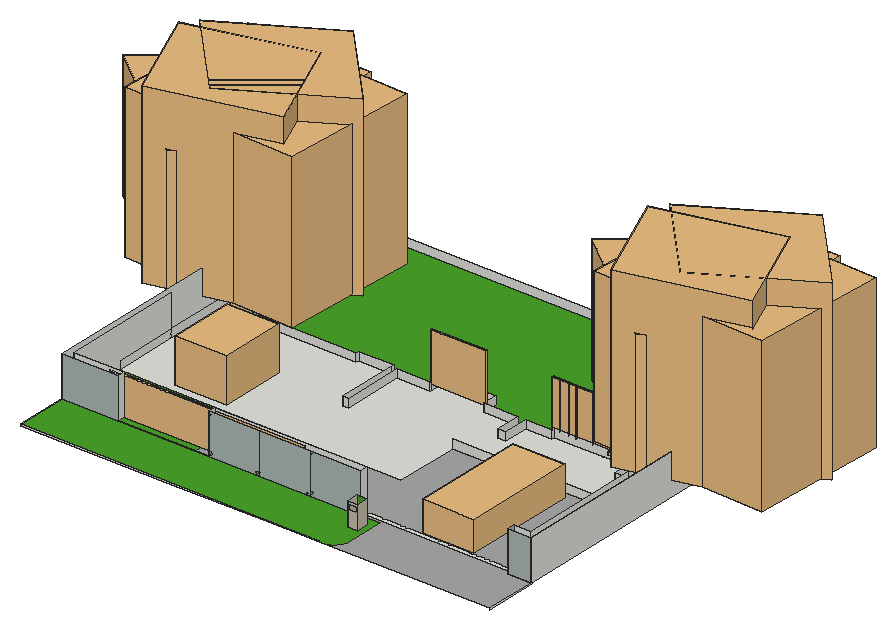
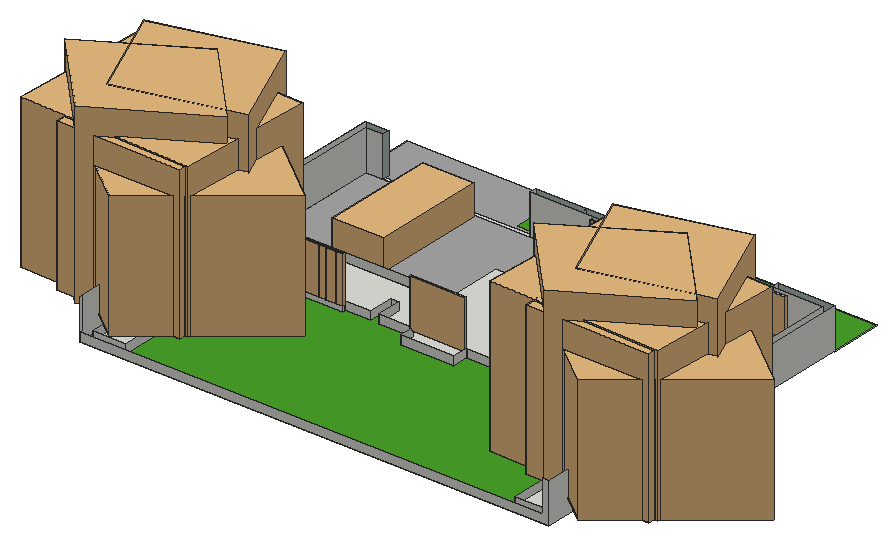
# SketchUp Ruby script. Lengths in inches.
U = 1.inch
M = Sketchup.active_model
def pt(a) = Geom::Point3d.new(a.map { |v| v * U })
def face(e, loops, mat)
  f = e.add_face(loops[0].map { |a| pt(a) })
  loops[1..].each { |l| e.add_face(l.map { |a| pt(a) }).erase! }
  f.material = f.back_material = mat if mat
  f
end
# faces: each face lists its corners as indices into pts; further lists are holes
def faces(e, pts, list, mat = nil) = list.each { |f| face(e, (f[0].is_a?(Array) ? f : [f]).map { |l| l.map { |i| pts[i] } }, mat) }
# xy, xz, yz: faces in a plane at the given z, y or x. An outline is a flat list of corners, or four numbers for a rectangle; further outlines are holes
def ring(l) = l.size == 4 ? [[l[0], l[1]], [l[2], l[1]], [l[2], l[3]], [l[0], l[3]]] : l.each_slice(2).to_a
def flat(e, list, mat, &to3) = list.each { |f| face(e, (f[0].is_a?(Array) ? f : [f]).map { |l| ring(l).map { |u, v| to3.(u, v) } }, mat) }
def xy(e, z, list, mat = nil) = flat(e, list, mat) { |x, y| [x, y, z] }
def xz(e, y, list, mat = nil) = flat(e, list, mat) { |x, z| [x, y, z] }
def yz(e, x, list, mat = nil) = flat(e, list, mat) { |y, z| [x, y, z] }
def lines(e, pts, list) = list.each { |a, b| e.add_line(pt(pts[a]), pt(pts[b])) }
# prism: a flat outline (further loops are holes) pulled along v
def prism(e, loops, v, mat = nil)
  f = face(e, loops, mat); d = Geom::Vector3d.new(v.map { |x| x * U })
  f.pushpull(f.normal.samedirection?(d) ? d.length : -d.length)
end
def box(e, o, s, mat = nil) = prism(e, [[o, [o[0] + s[0], o[1], o[2]], [o[0] + s[0], o[1] + s[1], o[2]], [o[0], o[1] + s[1], o[2]]]], [0, 0, s[2]], mat)
def at(x, y, z, deg = 0) = Geom::Transformation.translation(pt([x, y, z])) * Geom::Transformation.rotation(ORIGIN, Z_AXIS, deg.degrees)
def axes(o, x, y, z) = Geom::Transformation.new([*x, 0, *y, 0, *z, 0, *pt(o).to_a, 1])
def part(name) = M.definitions.add(name)
# library, detail: a bought-in or finely detailed component or shape, given as its bounding box
def library(name, o, s) = part(name).tap { |d| box(d.entities, o, s) }
def detail(e, o, s) = box(e.add_group.entities, o, s)
def put(e, d, t, mat = nil) = e.add_instance(d, t).tap { |i| i.material = mat if mat }
def group(e, t, mat = nil) = e.add_group.tap { |g| g.transformation = t; g.material = mat if mat }.entities
root = M.entities
M.materials.add("Material~3").color = [123, 113, 102]
M.materials.add("[0116_Lavender]").color = [73, 163, 41]
M.materials.add("[0132_LightGray]").color = [169, 169, 169]
M.materials.add("[Slate]").color = [172, 186, 182]
M.materials.add("[Tile Canvas]").color = [199, 192, 173]
M.materials.add("[Tile Grey]").color = [168, 168, 168]
c1 = library("Group\#65",[-33.32,-34.9375,32.67],[162.87,159.66,128.34])
c2 = library("Group\#81",[-10.45,-6.67,0],[121.7,116.61,164.95])
c3 = library("Group\#82",[-10.45,-6.67,0],[121.7,116.61,164.95])
c4 = library("Group\#69",[-10.45,-6.67,0],[121.7,116.61,164.95])
c5 = library("Group\#83",[-33.32,-34.9375,32.67],[162.87,159.66,128.34])
c6 = library("Group\#64",[-33.32,-34.9375,81.35],[162.87,159.66,79.66])
c7 = library("Group\#80",[-33.32,-34.9375,77.91],[162.87,159.66,83.1])
c8 = part("Palem Elek")
put(c8.entities,c1,axes([92.2,20.3,-29.73],[0.70711,0.70711,0],[-0.70711,0.70711,0],[0,0,0.91208]))
put(c8.entities,c2,axes([60.27,20.78,0],[1,0,0],[0,1,0],[0,0,0.85762]))
put(c8.entities,c3,at(25.45,60.83,0,-53.5))
put(c8.entities,c4,at(84.4375,135.48,0,-161.4))
put(c8.entities,c5,axes([38.54,105.7,-36.19],[-0.04013,-0.99919,0],[0.99919,-0.04013,0],[0,0,1.11001]))
put(c8.entities,c6,axes([57.15,96.51,-54.45],[-0.02003,-0.49872,0.02965],[0.4996,-0.02007,0],[0.00123,0.03065,0.51628]))
put(c8.entities,c7,axes([74.94,50.39,-54.06],[0.40095,0.29715,0.03075],[-0.29654,0.38966,0.10114],[0.04012,-0.11026,0.54246]))
c9 = part("palem elek\#1")
put(c9.entities,c8,at(-81.14,-74.56,-0.83))
c10 = part("Coqueiro")
put(c10.entities,c9,axes([83.17,89.39,9.5625],[0,1.1016,0],[-1.377,0,0],[0,0,1.39284]))
c11 = library("Potted broadleaf plant",[-29.7,0,-10.87],[31.67,38.52,72.45])
c12 = library("Sem+nome (1)",[20.77,3.52,-2.22],[96.42,122.82,82.56])
c13 = library("Sliding Gate",[0,0,0],[194.88,4.13,70.58])
c14 = library("3 door",[0,0,0],[74.8,3.9375,43.31])
c15 = library("3DGeom~4_Defintion",[362.52,-15.59,12.6],[288.85,70.11,1000])
c16 = library("BMW 8 Series M850i 2019",[-14.25,0.77,-0.16],[87.38,190.63,50.87])
xy(root,-10.51,[[836.67,498.28,1113.48,505.1],[[288.55,611.53,288.55,1146.63,352.17,1146.63,352.17,732.28,363.11,732.28,363.11,845.35,545.16,845.35,545.16,851.0625,610.53,851.0625,610.53,732.28,621.47,732.28,621.47,845.35,684.16,845.35,684.16,874.25,784.44,874.25,784.44,845.35,848.72,845.35,848.72,798.41,864.05,798.41,864.05,845.35,911.51,845.35,911.51,851.0625,1080.92,851.0625,1080.92,1146.63,1144.18,1146.63,1144.18,732.28,816.46,732.28,816.46,611.53],[1065.59,801.78,1080.92,845.35]]])
xy(root,-10.51,[[[276.92,393.78,847.17,393.78,850.2,394.71,853.13,395.9,855.95,397.35,858.62,399.04,861.14,400.97,863.47,403.1,865.61,405.44,867.53,407.96,869.23,410.63,870.67,413.45,871.87,416.38,872.8,419.41,872.8,491.47,836.67,491.47,836.67,505.1,551.82,505.1,551.82,491.47,382.82,491.47,382.82,505.1,288.55,505.1,288.55,1146.63,352.17,1146.63,352.17,732.28,363.11,732.28,363.11,845.35,545.16,845.35,545.16,851.0625,610.53,851.0625,610.53,732.28,621.47,732.28,621.47,845.35,684.16,845.35,684.16,874.25,784.44,874.25,784.44,845.35,848.72,845.35,848.72,798.41,864.05,798.41,864.05,845.35,911.51,845.35,911.51,851.0625,1080.92,851.0625,1080.92,1146.63,1144.18,1146.63,1144.18,505.1,1113.48,505.1,1113.48,491.47,1156.17,491.47,1156.17,1160.85,276.92,1160.85],[842.6875,453.42,861.125,475.99]],[382.82,491.47,526.25,491.47,531.46,611.53,288.55,611.53,288.55,505.1,382.82,505.1]],"[0116_Lavender]")
xy(root,-10.51,[[847.17,393.78,1156.17,393.78,1156.17,491.47,1113.48,491.47,1113.48,498.28,836.67,498.28,836.67,491.47,872.8,491.47,872.8,419.41,871.87,416.38,870.67,413.45,869.23,410.63,867.53,407.96,865.61,405.44,863.47,403.1,861.14,400.97,858.62,399.04,855.95,397.35,853.13,395.9,850.2,394.71],[526.25,491.47,551.82,491.47,551.82,505.1,1144.18,505.1,1144.18,732.28,816.46,732.28,816.46,611.53,531.46,611.53]],"[Tile Grey]")
xz(root,393.78,[[276.92,-12.6875,551.82,-12.6875,836.67,-10.51,276.92,-10.51]])
xz(root,453.42,[[[842.6875,-10.51,861.125,32.74],[845.04,19.53,859.16,29.34]]],"[Tile Canvas]")
xz(root,475.99,[[842.6875,-10.51,861.125,32.74]],"[0116_Lavender]")
xz(root,491.47,[[382.82,-12.6875,551.82,-10.51]])
xz(root,491.47,[[643.03,-7.89,643.52,-7.82,643.97,-7.63,644.36,-7.34,644.66,-6.95,644.85,-6.5,644.91,-6.01,644.85,-5.52,644.66,-5.07,644.36,-4.68,643.97,-4.39,643.52,-4.2,643.03,-4.14,642.55,-4.2,642.1,-4.39,641.71,-4.68,641.41,-5.07,641.22,-5.52,641.16,-6.01,641.22,-6.5,641.41,-6.95,641.71,-7.34,642.1,-7.63,642.55,-7.82],[737.99,-7.89,738.47,-7.82,738.92,-7.63,739.3125,-7.34,739.61,-6.95,739.8,-6.5,739.86,-6.01,739.8,-5.52,739.61,-5.07,739.3125,-4.68,738.92,-4.39,738.47,-4.2,737.99,-4.14,737.5,-4.2,737.05,-4.39,736.66,-4.68,736.36,-5.07,736.17,-5.52,736.11,-6.01,736.17,-6.5,736.36,-6.95,736.66,-7.34,737.05,-7.63,737.5,-7.82],[832.9375,-7.89,833.42,-7.82,833.875,-7.63,834.26,-7.34,834.56,-6.95,834.75,-6.5,834.8125,-6.01,834.75,-5.52,834.56,-5.07,834.26,-4.68,833.875,-4.39,833.42,-4.2,832.9375,-4.14,832.45,-4.2,832,-4.39,831.61,-4.68,831.3125,-5.07,831.125,-5.52,831.0625,-6.01,831.125,-6.5,831.3125,-6.95,831.61,-7.34,832,-7.63,832.45,-7.82],[555.3,-6.41,555.79,-6.4,556.26,-6.26,556.68,-6.01,557.02,-5.66,557.25,-5.23,557.37,-4.75,557.35,-4.26,557.22,-3.79,556.96,-3.375,556.61,-3.04,556.18,-2.8,555.7,-2.6875,555.21,-2.7,554.74,-2.84,554.32,-3.09,553.99,-3.45,553.75,-3.875,553.64,-4.35,553.65,-4.84,553.79,-5.31,554.04,-5.73,554.4,-6.07,554.83,-6.3],[650.25,-6.41,650.74,-6.4,651.21,-6.26,651.63,-6.01,651.97,-5.66,652.2,-5.23,652.32,-4.75,652.3,-4.26,652.17,-3.79,651.91,-3.375,651.56,-3.04,651.13,-2.8,650.65,-2.6875,650.16,-2.7,649.69,-2.84,649.27,-3.09,648.9375,-3.45,648.7,-3.875,648.59,-4.35,648.6,-4.84,648.74,-5.31,648.99,-5.73,649.35,-6.07,649.78,-6.3],
  [745.2,-6.41,745.69,-6.4,746.16,-6.26,746.58,-6.01,746.92,-5.66,747.15,-5.23,747.27,-4.75,747.26,-4.26,747.12,-3.79,746.86,-3.375,746.51,-3.04,746.08,-2.8,745.6,-2.6875,745.11,-2.7,744.64,-2.84,744.23,-3.09,743.89,-3.45,743.65,-3.875,743.54,-4.35,743.55,-4.84,743.6875,-5.31,743.94,-5.73,744.3,-6.07,744.73,-6.3]],"[0132_LightGray]")
xz(root,491.47,[[276.92,-12.6875,382.82,65.1875],[[551.82,-12.6875,836.67,-10.51,836.67,65.1875,551.82,65.1875],[643.03,-7.89,642.55,-7.82,642.1,-7.63,641.71,-7.34,641.41,-6.95,641.22,-6.5,641.16,-6.01,641.22,-5.52,641.41,-5.07,641.71,-4.68,642.1,-4.39,642.55,-4.2,643.03,-4.14,643.52,-4.2,643.97,-4.39,644.36,-4.68,644.66,-5.07,644.85,-5.52,644.91,-6.01,644.85,-6.5,644.66,-6.95,644.36,-7.34,643.97,-7.63,643.52,-7.82],[737.99,-7.89,737.5,-7.82,737.05,-7.63,736.66,-7.34,736.36,-6.95,736.17,-6.5,736.11,-6.01,736.17,-5.52,736.36,-5.07,736.66,-4.68,737.05,-4.39,737.5,-4.2,737.99,-4.14,738.47,-4.2,738.92,-4.39,739.3125,-4.68,739.61,-5.07,739.8,-5.52,739.86,-6.01,739.8,-6.5,739.61,-6.95,739.3125,-7.34,738.92,-7.63,738.47,-7.82],[643.03,57.74,642.55,57.8,642.1,57.99,641.71,58.29,641.41,58.68,641.22,59.13,641.16,59.61,641.22,60.1,641.41,60.55,641.71,60.94,642.1,61.24,642.55,61.43,643.03,61.49,643.52,61.43,643.97,61.24,644.36,60.94,644.66,60.55,644.85,60.1,644.91,59.61,644.85,59.13,644.66,58.68,644.36,58.29,643.97,57.99,643.52,57.8],[737.99,57.74,737.5,57.8,737.05,57.99,736.66,58.29,736.36,58.68,736.17,59.13,736.11,59.61,736.17,60.1,736.36,60.55,736.66,60.94,737.05,61.24,737.5,61.43,737.99,61.49,738.47,61.43,738.92,61.24,739.3125,60.94,739.61,60.55,739.8,60.1,739.86,59.61,739.8,59.13,739.61,58.68,739.3125,58.29,738.92,57.99,738.47,57.8],[832.9375,-7.89,832.45,-7.82,832,-7.63,831.61,-7.34,831.3125,-6.95,831.125,-6.5,831.0625,-6.01,831.125,-5.52,831.3125,-5.07,831.61,-4.68,832,-4.39,832.45,-4.2,832.9375,-4.14,833.42,-4.2,833.875,-4.39,834.26,-4.68,834.56,-5.07,834.75,-5.52,834.8125,-6.01,834.75,-6.5,834.56,-6.95,834.26,-7.34,833.875,-7.63,833.42,-7.82],[832.9375,57.74,832.45,57.8,832,57.99,831.61,58.29,831.3125,58.68,831.125,59.13,831.0625,59.61,831.125,60.1,831.3125,60.55,831.61,60.94,832,61.24,832.45,61.43,832.9375,61.49,833.42,61.43,833.875,61.24,834.26,60.94,834.56,60.55,834.75,60.1,834.8125,59.61,834.75,59.13,834.56,58.68,834.26,58.29,833.875,57.99,833.42,57.8],[650.25,59.21,649.78,59.33,649.35,59.56,648.99,59.9,648.74,60.32,648.6,60.78,648.59,61.27,648.7,61.75,648.9375,62.18,649.27,62.53,649.69,62.79,650.16,62.93,650.65,62.9375,651.13,62.82,651.56,62.59,651.91,62.25,652.17,61.83,652.3,61.36,652.32,60.875,652.2,60.4,651.97,59.97,651.63,59.61,651.21,59.36,650.74,59.22],[745.2,59.21,744.73,59.33,744.3,59.56,743.94,59.9,743.6875,60.32,743.55,60.78,743.54,61.27,743.65,61.75,743.89,62.18,744.23,62.53,744.64,62.79,745.11,62.93,745.6,62.9375,746.08,62.82,746.51,62.59,746.86,62.25,747.12,61.83,747.26,61.36,747.27,60.875,747.15,60.4,746.92,59.97,746.58,59.61,746.16,59.36,745.69,59.22],[555.3,-6.41,554.83,-6.3,554.4,-6.07,554.04,-5.73,553.79,-5.31,553.65,-4.84,553.64,-4.35,553.75,-3.875,553.99,-3.45,554.32,-3.09,554.74,-2.84,555.21,-2.7,555.7,-2.6875,556.18,-2.8,556.61,-3.04,556.96,-3.375,557.22,-3.79,557.35,-4.26,557.37,-4.75,557.25,-5.23,557.02,-5.66,556.68,-6.01,556.26,-6.26,555.79,-6.4],[650.25,-6.41,649.78,-6.3,649.35,-6.07,648.99,-5.73,648.74,-5.31,648.6,-4.84,648.59,-4.35,648.7,-3.875,648.9375,-3.45,649.27,-3.09,649.69,-2.84,650.16,-2.7,650.65,-2.6875,651.13,-2.8,651.56,-3.04,651.91,-3.375,652.17,-3.79,652.3,-4.26,652.32,-4.75,652.2,-5.23,651.97,-5.66,651.63,-6.01,651.21,-6.26,650.74,-6.4],[745.2,-6.41,744.73,-6.3,744.3,-6.07,743.94,-5.73,743.6875,-5.31,743.55,-4.84,743.54,-4.35,743.65,-3.875,743.89,-3.45,744.23,-3.09,744.64,-2.84,745.11,-2.7,745.6,-2.6875,746.08,-2.8,746.51,-3.04,746.86,-3.375,747.12,-3.79,747.26,-4.26,747.27,-4.75,747.15,-5.23,746.92,-5.66,746.58,-6.01,746.16,-6.26,745.69,-6.4],[555.3,59.21,554.83,59.33,554.4,59.56,554.04,59.9,553.79,60.32,553.65,60.78,553.64,61.27,553.75,61.75,553.99,62.18,554.32,62.53,554.74,62.79,555.21,62.93,555.7,62.9375,556.18,62.82,556.61,62.59,556.96,62.25,557.22,61.83,557.35,61.36,557.37,60.875,557.25,60.4,557.02,59.97,556.68,59.61,556.26,59.36,555.79,59.22]],[1113.48,-10.51,1156.17,65.1875]],"[Slate]")
xz(root,505.1,[[288.55,-10.51,382.82,65.1875],[551.82,-10.51,836.67,65.1875],[1113.48,-10.51,1144.18,65.1875]])
xz(root,732.28,[[352.17,-10.51,363.11,5.1875],[610.53,-10.51,621.47,5.1875],[816.46,-10.51,1144.18,5.1875]])
xz(root,798.41,[[848.72,-10.51,864.05,5.1875]])
xz(root,801.78,[[1065.59,-10.51,1080.92,5.1875]])
xz(root,845.35,[[363.11,-10.51,545.16,5.1875],[621.47,-10.51,684.16,5.1875],[784.44,-10.51,848.72,5.1875],[864.05,-10.51,911.51,5.1875],[1065.59,-10.51,1080.92,5.1875],
  [1016.125,-0.125,1065.59,5.1875]])
xz(root,851.0625,[[545.16,-10.51,610.53,5.1875],[911.51,-10.51,1016.125,5.1875],[1016.125,-10.51,1075.21,5.1875],[1075.21,-10.51,1080.92,5.1875]])
xz(root,874.25,[[684.16,-10.51,784.44,5.1875]])
xz(root,1146.63,[[288.55,-10.51,352.17,5.1875],[1080.92,-10.51,1144.18,5.1875]])
xz(root,1160.85,[[276.92,-10.51,276.92,65.1875,288.55,65.1875,288.55,5.1875,1156.17,5.1875,1156.17,-10.51]])
yz(root,276.92,[[393.78,-12.6875,491.47,-10.51],[491.47,-10.51,1160.85,65.1875]])
yz(root,288.55,[[505.1,-10.51,611.53,-10.51,611.53,5.1875,732.28,5.1875,732.28,65.1875,505.1,65.1875],[611.53,-10.51,732.28,5.1875],[732.28,-10.51,1146.63,5.1875]])
yz(root,352.17,[[732.28,-10.51,1146.63,5.1875]])
yz(root,363.11,[[732.28,-10.51,845.35,5.1875]])
yz(root,382.82,[[491.47,-10.51,505.1,65.1875]])
yz(root,545.16,[[845.35,-10.51,851.0625,5.1875]])
yz(root,551.82,[[491.47,-10.51,505.1,65.1875]])
yz(root,610.53,[[732.28,-10.51,846.1,5.1875],[846.1,-10.51,851.0625,5.1875]])
yz(root,621.47,[[732.28,-10.51,845.35,5.1875]])
yz(root,684.16,[[845.35,-10.51,846.1,5.1875],[846.1,-10.51,874.25,5.1875]])
yz(root,784.44,[[845.35,-10.51,846.1,5.1875],[846.1,-10.51,874.25,5.1875]])
yz(root,836.67,[[491.47,-10.51,505.1,65.1875]])
yz(root,842.6875,[[453.42,-10.51,475.99,32.74]],"[Tile Canvas]")
yz(root,848.72,[[798.41,-10.51,845.35,5.1875]])
yz(root,861.125,[[453.42,-10.51,475.99,32.74]],"[Tile Canvas]")
yz(root,864.05,[[798.41,-10.51,845.35,5.1875]])
yz(root,911.51,[[845.35,-10.51,846.1,5.1875],[846.1,-10.51,851.0625,5.1875]])
yz(root,1016.125,[[845.35,-0.125,851.0625,5.1875]])
yz(root,1065.59,[[801.78,-10.51,845.35,5.1875]])
yz(root,1080.92,[[801.78,-10.51,845.35,5.1875],[851.0625,-10.51,1146.63,5.1875]])
yz(root,1113.48,[[491.47,-10.51,505.1,65.1875]],"[Slate]")
yz(root,1144.18,[[505.1,-10.51,732.28,65.1875],[732.28,-10.51,1146.63,5.1875]])
yz(root,1156.17,[[491.47,-10.51,1160.85,-10.51,1160.85,5.1875,1155.13,5.1875,1155.13,65.1875,491.47,65.1875]])
yz(root,1156.87,[[393.78,-12.6875,491.47,-10.51],[491.47,-10.51,1160.85,65.1875]])
p = [[646.77,491.47,65.1875],[646.77,491.47,-10.51],[741.72,491.47,65.1875],[741.72,491.47,-10.51]]
lines(root,p,[[0,1],[2,3]])
put(root,c10,axes([127.53,830.17,6.32],[1.44,0,0],[0,1.44,0],[0,0,1.44]))
put(root,c11,axes([357.81,858.27,6.22],[2,0,0],[0,2,0],[0,0,2]))
put(root,c11,axes([357.81,924.09,6.22],[2,0,0],[0,2,0],[0,0,2]))
put(root,c12,at(368.94,611.53,-0.125))
put(root,c13,axes([355.375,505.1,-10.51],[1.88,0,0],[0,1,0],[0,0,1]))
put(root,c14,axes([684.16,846.14,1.53],[1.37387,0,0],[0,0.86071,0],[0,0,2.11056]))
put(root,c15,axes([867.8,854.26,0.98],[0.11056,0,0],[0,-0.05859,0],[0,0,0.08734]),"Material~3")
put(root,c15,axes([881.84,854.26,0.98],[0.11056,0,0],[0,-0.05859,0],[0,0,0.08734]),"Material~3")
put(root,c15,axes([912.42,854.26,0.98],[0.11056,0,0],[0,-0.05859,0],[0,0,0.08734]),"Material~3")
put(root,c16,axes([1020.16,720.81,-10.33],[-1.11,0,0],[0,-1.11,0],[0,0,1.11]))
put(root,c15,axes([944.11,854.26,0.98],[0.11056,0,0],[0,-0.05859,0],[0,0,0.08734]),"Material~3")
put(root,c10,axes([1007.47,830.17,6.32],[1.44,0,0],[0,1.44,0],[0,0,1.44]))
